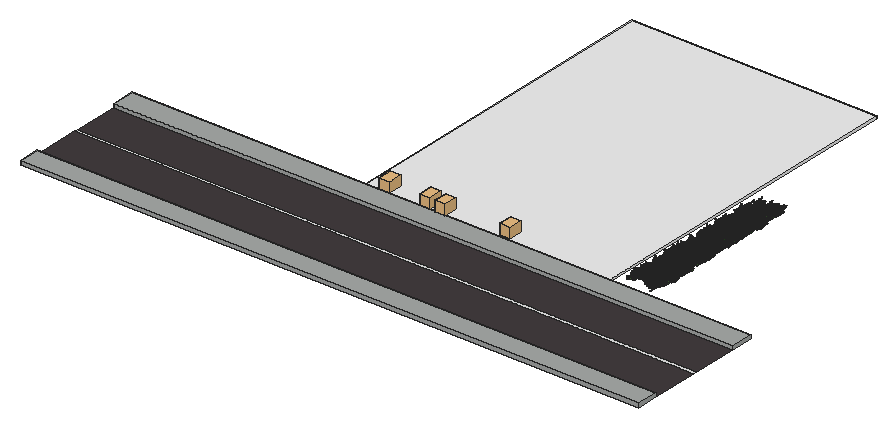
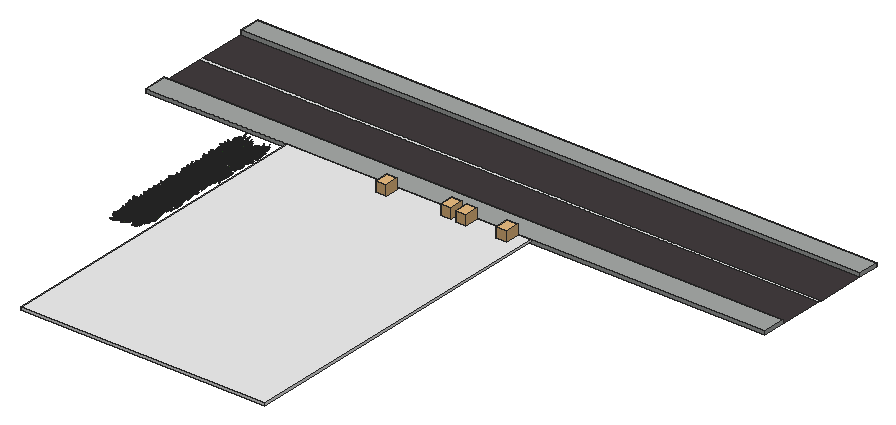
# SketchUp Ruby script. Lengths in inches.
U = 1.inch
M = Sketchup.active_model
def pt(a) = Geom::Point3d.new(a.map { |v| v * U })
def face(e, loops, mat)
  f = e.add_face(loops[0].map { |a| pt(a) })
  loops[1..].each { |l| e.add_face(l.map { |a| pt(a) }).erase! }
  f.material = f.back_material = mat if mat
  f
end
# faces: each face lists its corners as indices into pts; further lists are holes
def faces(e, pts, list, mat = nil) = list.each { |f| face(e, (f[0].is_a?(Array) ? f : [f]).map { |l| l.map { |i| pts[i] } }, mat) }
# xy, xz, yz: faces in a plane at the given z, y or x. An outline is a flat list of corners, or four numbers for a rectangle; further outlines are holes
def ring(l) = l.size == 4 ? [[l[0], l[1]], [l[2], l[1]], [l[2], l[3]], [l[0], l[3]]] : l.each_slice(2).to_a
def flat(e, list, mat, &to3) = list.each { |f| face(e, (f[0].is_a?(Array) ? f : [f]).map { |l| ring(l).map { |u, v| to3.(u, v) } }, mat) }
def xy(e, z, list, mat = nil) = flat(e, list, mat) { |x, y| [x, y, z] }
def xz(e, y, list, mat = nil) = flat(e, list, mat) { |x, z| [x, y, z] }
def yz(e, x, list, mat = nil) = flat(e, list, mat) { |y, z| [x, y, z] }
def lines(e, pts, list) = list.each { |a, b| e.add_line(pt(pts[a]), pt(pts[b])) }
# prism: a flat outline (further loops are holes) pulled along v
def prism(e, loops, v, mat = nil)
  f = face(e, loops, mat); d = Geom::Vector3d.new(v.map { |x| x * U })
  f.pushpull(f.normal.samedirection?(d) ? d.length : -d.length)
end
def box(e, o, s, mat = nil) = prism(e, [[o, [o[0] + s[0], o[1], o[2]], [o[0] + s[0], o[1] + s[1], o[2]], [o[0], o[1] + s[1], o[2]]]], [0, 0, s[2]], mat)
def at(x, y, z, deg = 0) = Geom::Transformation.translation(pt([x, y, z])) * Geom::Transformation.rotation(ORIGIN, Z_AXIS, deg.degrees)
def axes(o, x, y, z) = Geom::Transformation.new([*x, 0, *y, 0, *z, 0, *pt(o).to_a, 1])
def part(name) = M.definitions.add(name)
# library, detail: a bought-in or finely detailed component or shape, given as its bounding box
def library(name, o, s) = part(name).tap { |d| box(d.entities, o, s) }
def detail(e, o, s) = box(e.add_group.entities, o, s)
def put(e, d, t, mat = nil) = e.add_instance(d, t).tap { |i| i.material = mat if mat }
def group(e, t, mat = nil) = e.add_group.tap { |g| g.transformation = t; g.material = mat if mat }.entities
root = M.entities
M.materials.add("Material10").color = [48, 90, 38]
M.materials.add("Material11").color = [68, 110, 48]
M.materials.add("Material12").color = [48, 90, 48]
M.materials.add("Material13").color = [58, 110, 58]
M.materials.add("Material14").color = [58, 90, 38]
M.materials.add("Material15").color = [68, 100, 58]
M.materials.add("Material16").color = [48, 100, 38]
M.materials.add("Material9").color = [68, 110, 58]
M.materials.add("Tiles Marble White 03 180cm\#1").color = [241, 241, 241]
M.materials.add("[Asphalt_New]").color = [67, 60, 62]
M.materials.add("[Color_001]1").color = [226, 226, 226]
M.materials.add("[Concrete_Form_4x8]").color = [167, 170, 168]
c1 = library("Plant 260 031 02",[-5.66,-10.61,-5.67],[17.04,23.05,21.91])
c2 = part("组\#1")
xy(c2.entities,0,[[37.85,0,110.93,506],[116.54,0,195.23,506]],"[Asphalt_New]")
xy(c2.entities,0,[[110.93,0,116.54,506]],"[Color_001]1")
xy(c2.entities,6.25,[[0,0,37.85,506],[195.23,0,229.75,506]],"[Concrete_Form_4x8]")
xz(c2.entities,0,[[0,0,37.85,6.25],[195.23,0,229.75,6.25]],"[Concrete_Form_4x8]")
xz(c2.entities,506,[[0,0,37.85,6.25],[195.23,0,229.75,6.25]],"[Concrete_Form_4x8]")
yz(c2.entities,0,[[0,0,506,6.25]],"[Concrete_Form_4x8]")
yz(c2.entities,37.85,[[0,0,506,6.25]],"[Concrete_Form_4x8]")
yz(c2.entities,195.23,[[0,0,506,6.25]],"[Concrete_Form_4x8]")
yz(c2.entities,229.75,[[0,0,506,6.25]],"[Concrete_Form_4x8]")
c3 = part("grass00")
p = [[-0.6875,0.15,0],[-0.56,0.08,5.52],[-0.04,0.03,2.76],[0.48,-0.02,0],[0.35,-0.02,5.52],[-0.1,-0.14,5.52],
  [-0.12,0.65,8.37],[-0.42,0.65,8.37]]
faces(c3.entities,p,[[0,1,2,3],[3,2,4],[1,5,2],[5,4,2],[1,6,5],[4,5,6],[7,6,1]])
c4 = part("Group16\#1")
put(c4.entities,c3,axes([1.44,-0.61,-0.01],[0.05352,0.12609,0],[-0.10704,0.04543,0.07239],[0.06664,-0.02828,0.11628]),"Material12")
put(c4.entities,c3,axes([0.76,-0.15,-0.01],[0.04676,0.24062,0],[-0.23162,0.04501,0.06642],[0.0652,-0.01267,0.23595]),"Material9")
put(c4.entities,c3,axes([0.79,0.01,-0.01],[-0.00606,0.34651,0],[-0.34381,-0.00602,0.0432],[0.04319,0.00076,0.34386]))
put(c4.entities,c3,axes([1,0.23,-0.01],[-0.07192,0.31144,0],[-0.28722,-0.06632,0.1236],[0.12043,0.02781,0.29478]),"Material11")
put(c4.entities,c3,axes([1.66,0.77,-0.01],[-0.13828,0.29651,0],[-0.21551,-0.1005,0.22471],[0.20365,0.09498,0.23779]),"Material16")
put(c4.entities,c3,axes([0.6875,0.52,-0.01],[-0.18126,0.24051,0],[-0.22746,-0.17142,0.09788],[0.07817,0.05891,0.28481]),"Material11")
put(c4.entities,c3,axes([0.68,0.78,-0.01],[-0.215,0.18688,0],[-0.12385,-0.14248,0.21334],[0.13995,0.16101,0.18878]),"Material9")
put(c4.entities,c3,axes([0.56,1,-0.01],[-0.13756,0.07624,0],[-0.06159,-0.11112,0.0927],[0.04494,0.08108,0.12705]),"Material11")
put(c4.entities,c3,axes([0.2,0.64,-0.01],[-0.23729,0.07254,0],[-0.05711,-0.18681,0.153],[0.04473,0.14632,0.19535]),"Material16")
put(c4.entities,c3,axes([0.0625,0.72,-0.01],[-0.28874,0.02525,0],[-0.02179,-0.24916,0.14647],[0.01276,0.14591,0.25012]),"Material9")
put(c4.entities,c3,axes([-0.08,0.62,-0.01],[-0.34089,-0.04187,0],[0.03255,-0.26504,0.216],[-0.02633,0.21439,0.26703]),"Material16")
put(c4.entities,c3,axes([-0.34,0.98,-0.01],[-0.14314,-0.0493,0],[0.04397,-0.12769,0.06843],[-0.02228,0.0647,0.13505]),"Material16")
put(c4.entities,c3,axes([-0.87,1.45,-0.01],[-0.23488,-0.14114,0],[0.13761,-0.22901,0.06087],[-0.03135,0.05217,0.26717]))
put(c4.entities,c3,axes([-0.72,0.77,-0.01],[-0.14208,-0.13251,0],[0.07209,-0.0773,0.16301],[-0.11118,0.11922,0.1057]),"Material16")
put(c4.entities,c3,axes([-0.62,0.43,-0.01],[-0.14845,-0.21203,0],[0.18654,-0.13061,0.12304],[-0.10079,0.07057,0.22772]),"Material9")
put(c4.entities,c3,axes([-0.68,0.29,-0.01],[-0.13639,-0.32136,0],[0.31723,-0.13464,0.05579],[-0.05136,0.0218,0.34462]),"Material10")
put(c4.entities,c3,axes([-0.64,0.125,-0.01],[-0.0458,-0.23569,0],[0.22124,-0.043,0.08276],[-0.08124,0.01579,0.22538]),"Material13")
put(c4.entities,c3,axes([-1.6,-0.03,-0.01],[0.00576,-0.32897,0],[0.27526,0.00482,0.18018],[-0.18015,-0.00315,0.2753]),"Material11")
put(c4.entities,c3,axes([-1.36,-0.31,-0.01],[0.05718,-0.24765,0],[0.18172,0.04196,0.17267],[-0.16825,-0.03885,0.1865]),"Material16")
put(c4.entities,c3,axes([-1.54,-0.72,-0.01],[0.06537,-0.14017,0],[0.13555,0.06321,0.03939],[-0.0357,-0.01665,0.14956]))
put(c4.entities,c3,axes([-1.19,-0.9,-0.01],[0.09597,-0.12735,0],[0.11214,0.08451,0.07557],[-0.06035,-0.04548,0.14042]),"Material15")
put(c4.entities,c3,axes([-0.47,-0.54,-0.01],[0.11588,-0.10072,0],[0.0618,0.0711,0.12124],[-0.07953,-0.0915,0.0942]))
put(c4.entities,c3,axes([-0.47,-0.84,-0.01],[0.11927,-0.0661,0],[0.06603,0.11913,0.00646],[-0.00313,-0.00565,0.13621]),"Material11")
put(c4.entities,c3,axes([-0.38,-1.24,-0.01],[0.28037,-0.08571,0],[0.0618,0.20215,0.20315],[-0.05939,-0.19428,0.21139]),"Material15")
put(c4.entities,c3,axes([-0.06,-0.66,-0.01],[0.22719,-0.01987,0],[0.01247,0.14255,0.17758],[-0.01547,-0.17691,0.1431]),"Material14")
put(c4.entities,c3,axes([0.11,-0.89,-0.01],[0.14882,0.01828,0],[-0.01058,0.08611,0.12229],[0.01491,-0.12138,0.08676]),"Material12")
put(c4.entities,c3,axes([0.25,-0.72,-0.01],[0.20481,0.07053,0],[-0.06206,0.18022,0.10291],[0.03351,-0.0973,0.1906]),"Material12")
put(c4.entities,c3,axes([0.85,-1.42,-0.01],[0.16481,0.09904,0],[-0.09472,0.15762,0.05616],[0.02893,-0.04814,0.18389]),"Material11")
put(c4.entities,c3,axes([1.01,-1.09,-0.01],[0.21858,0.20385,0],[-0.17495,0.1876,0.15339],[0.10462,-0.11218,0.25652]),"Material16")
put(c4.entities,c3,axes([1.01,-0.71,-0.01],[0.08733,0.12473,0],[-0.06445,0.04512,0.13037],[0.1068,-0.07477,0.07867]),"Material12")
c5 = part("Group15\#1")
put(c5.entities,c4,at(0,0,0))
c6 = part("3darcstudiotree_grass00\#1")
put(c6.entities,c5,at(0,0,0))
put(root,c1,at(411.73,241.75,16.75))
put(root,c1,at(479.07,241.3,16.75))
put(root,c1,at(505.1,239.68,16.75))
put(root,c2,axes([0,229.75,10.5],[0,-1,0],[2.0148,0,0],[0,0,1]))
g1 = group(root,at(420.73,303.57,12.75))
box(g1,[-36,-73.82,0],[402,549.37,4],"Tiles Marble White 03 180cm\#1")
put(root,c1,at(607.78,244.29,16.75))
put(root,c6,axes([800.67,339.93,12.99],[-0.98849,-6.07727,0],[3.06022,-2.60089,-0.02925],[0.10433,-0.08867,1.7044]))
put(root,c6,axes([800.7,291.18,12.99],[-3.25842,-2.83889,0],[0.88861,-5.32937,-0.04688],[0.07754,-0.46503,1.58936]))
put(root,c6,axes([800.98,446.97,12.99],[-1.08167,-7.23461,0],[2.82341,-2.20577,-0.03013],[0.10703,-0.08362,1.53631]))
put(root,c6,axes([800.78,348.7,12.99],[-1.3715,5.90605,0],[-2.459,-2.98374,-0.02935],[-0.08981,-0.10898,1.32321]))
put(root,c6,axes([800.82,311.72,12.99],[2.39933,-0.88558,0],[0.42391,6.00129,-0.03713],[0.0226,0.31997,1.39317]))
put(root,c6,axes([801.01,271.4,12.99],[1.11384,7.00141,0],[-2.3963,1.99197,-0.03897],[-0.1605,0.13341,1.53286]))
put(root,c6,axes([802.48,486.76,12.99],[0.27051,-7.1157,0],[3.04279,0.60444,-0.03115],[0.11632,0.02311,1.5702]))
put(root,c6,axes([803.05,273.92,12.99],[1.68247,-4.28756,0],[2.47865,5.08226,-0.03873],[0.1199,0.24584,1.89965]))
put(root,c6,axes([803.99,418.8,12.99],[1.17417,-7.15261,0],[2.37757,2.03942,-0.02337],[0.10494,0.09002,1.67088]))
put(root,c6,axes([803.49,282.77,12.99],[0.14761,6.20223,0],[-2.49222,0.30993,-0.03311],[-0.1396,0.01736,1.44579]))
put(root,c6,axes([804.68,413.44,12.99],[-2.29924,4.62436,0],[-1.90032,-4.937,-0.02195],[-0.06693,-0.17388,1.82186]))
put(root,c6,axes([805.44,366.33,12.99],[-2.97813,-1.40056,0],[0.64267,-7.14054,-0.02294],[0.01821,-0.20232,1.72347]))
put(root,c6,axes([804.71,346.85,12.99],[2.49242,-3.45573,0],[1.7696,6.66902,-0.03972],[0.07236,0.27271,1.6444]))
put(root,c6,axes([804.3,395.07,12.99],[2.7147,4.27072,0],[-1.80498,5.99513,-0.05897],[-0.14635,0.48608,1.91169]))
put(root,c6,axes([805.35,357.75,12.99],[-2.03898,5.04396,0],[-2.47769,-5.23352,-0.01856],[-0.05439,-0.11488,1.84646]))
put(root,c6,axes([805.07,262.63,12.99],[2.98145,-0.50513,0],[0.21055,6.4935,-0.02045],[0.00697,0.21501,1.8024]))
put(root,c6,axes([806.57,467.15,12.99],[-0.75501,-6.88565,0],[2.48437,-1.4234,-0.0349],[0.17754,-0.10172,1.84282]))
put(root,c6,axes([807.58,414.25,12.99],[-1.68018,-4.94064,0],[2.1447,-3.81105,-0.04864],[0.19458,-0.34576,1.88819]))
put(root,c6,axes([807.57,335.99,12.99],[-0.20197,-5.97763,0],[2.99307,-0.52842,-0.04603],[0.17968,-0.03172,1.61216]))
put(root,c6,axes([807.93,424.48,12.99],[-3.12761,-0.88156,0],[0.3332,-6.17695,-0.03319],[0.01691,-0.31352,1.55524]))
put(root,c6,axes([808.16,484.11,12.99],[-0.99694,-6.52822,0],[3.15637,-2.51865,-0.05387],[0.16231,-0.12952,1.46363]))
put(root,c6,axes([807.17,373.95,12.99],[2.63554,-0.55768,0],[0.2785,6.87733,-0.05657],[0.01882,0.46468,1.49576]))
put(root,c6,axes([808.32,438,12.99],[-2.32089,-3.24237,0],[1.49534,-5.59289,-0.04274],[0.09418,-0.35224,1.66217]))
put(root,c6,axes([807.77,448.18,12.99],[-0.45873,6.51223,0],[-2.66489,-0.98087,-0.03829],[-0.17369,-0.06393,1.70109]))
put(root,c6,axes([808.8,402.28,12.99],[-0.66116,-7.15231,0],[3.12813,-1.51095,-0.02196],[0.08817,-0.04259,1.79942]))
put(root,c6,axes([809.1,359.21,12.99],[-3.21408,-1.17783,0],[0.46153,-6.58082,-0.05495],[0.03492,-0.49786,1.60563]))
put(root,c6,axes([808.84,503.35,12.99],[1.24877,-5.5627,0],[2.72354,3.19474,-0.0206],[0.07656,0.08981,1.75423]))
put(root,c6,axes([808.12,349.19,12.99],[1.31042,5.62084,0],[-2.40949,2.93521,-0.05193],[-0.22679,0.27628,1.85357]))
put(root,c6,axes([809.27,427.29,12.99],[0.39081,-6.30576,0],[2.59761,0.84122,-0.02485],[0.13497,0.04371,1.97391]))
put(root,c6,axes([809.24,289.6,12.99],[-1.24855,7.36062,0],[-2.95077,-2.61536,-0.03012],[-0.11789,-0.10449,1.82227]))
put(root,c6,axes([809.14,475.84,12.99],[1.94397,4.23046,0],[-2.00085,4.80421,-0.04733],[-0.10808,0.2595,1.31836]))
put(root,c6,axes([809.4,315.22,12.99],[1.81122,6.51683,0],[-2.34506,3.4056,-0.05376],[-0.20203,0.2934,1.69687]))
put(root,c6,axes([810.82,299.03,12.99],[-2.35732,-4.30403,0],[1.59602,-4.56758,-0.04095],[0.12835,-0.36732,1.76156]))
put(root,c6,axes([811.1,441.46,12.99],[-1.06173,6.81827,0],[-2.83321,-2.30528,-0.05045],[-0.18809,-0.15304,1.63245]))
put(root,c6,axes([810.82,448.49,12.99],[1.33722,6.52276,0],[-2.56931,2.75228,-0.0367],[-0.17016,0.18228,1.99296]))
put(root,c6,axes([811.93,272.2,12.99],[-2.43072,-0.26359,0],[0.12868,-6.20017,-0.03298],[0.00788,-0.37965,1.87797]))
put(root,c6,axes([812.05,486.26,12.99],[-0.28872,-6.59919,0],[3.07918,-0.70393,-0.04439],[0.1451,-0.03317,1.39437]))
put(root,c6,axes([812.05,372.78,12.99],[-2.52267,-1.45098,0],[0.6301,-5.72418,-0.02412],[0.0269,-0.24434,1.61843]))
put(root,c6,axes([811.96,408.8,12.99],[-2.43865,3.44906,0],[-1.64275,-6.06912,-0.03047],[-0.05197,-0.19201,1.38852]))
put(root,c6,axes([811.48,479.91,12.99],[3.0655,-2.19528,0],[0.96462,7.03842,-0.0458],[0.05493,0.40081,1.7756]))
put(root,c6,axes([811.24,286.83,12.99],[2.42292,5.76115,0],[-1.8644,4.09707,-0.03508],[-0.11405,0.25063,1.59982]))
put(root,c6,axes([812.07,278.9375,12.99],[1.67096,-5.47383,0],[2.37534,3.78884,-0.05108],[0.18896,0.3014,1.79238]))
put(root,c6,axes([811.78,429.89,12.99],[-1.17862,5.63021,0],[-2.88982,-3.16101,-0.03408],[-0.09497,-0.10388,1.35762]))
put(root,c6,axes([812.84,418.5625,12.99],[-0.22622,-6.9338,0],[3.33092,-0.56785,-0.02024],[0.08123,-0.01385,1.84439]))
put(root,c6,axes([812.42,495.47,12.99],[2.21202,-5.60133,0],[2.54118,5.24369,-0.0538],[0.11673,0.24088,1.37259]))
put(root,c6,axes([812.81,344.54,12.99],[-1.98571,5.23753,0],[-2.13766,-4.2348,-0.03703],[-0.1146,-0.22703,1.58908]))
put(root,c6,axes([812.24,456.87,12.99],[0.79567,6.14666,0],[-3.11802,2.10902,-0.04809],[-0.14133,0.0956,1.36712]))
put(root,c6,axes([813.4,394.8,12.99],[2.47868,-2.12288,0],[0.90034,5.49294,-0.02122],[0.03978,0.2427,1.88089]))
put(root,c6,axes([814.86,448.8,12.99],[-2.3446,-1.56119,0],[0.96027,-7.5355,-0.03129],[0.03426,-0.26886,1.8441]))
put(root,c6,axes([815.66,289.4,12.99],[-2.01079,-4.32886,0],[2.15818,-5.23823,-0.03536],[0.10109,-0.24536,1.8008]))
put(root,c6,axes([814.9,368.54,12.99],[-0.72251,7.60275,0],[-2.80101,-1.39088,-0.03052],[-0.10543,-0.05235,1.38983]))
put(root,c6,axes([814.87,410.37,12.99],[-0.62691,6.10742,0],[-2.93793,-1.57578,-0.03302],[-0.11697,-0.06274,1.5061]))
put(root,c6,axes([815.87,284.22,12.99],[1.28541,-7.35574,0],[2.62364,2.39566,-0.05078],[0.21024,0.19197,1.72798]))
put(root,c6,axes([815.28,271.93,12.99],[0.93965,5.53656,0],[-2.59756,2.30353,-0.02781],[-0.10678,0.09469,1.57422]))
put(root,c6,axes([815.47,317.37,12.99],[2.51332,0.19657,0],[-0.11442,7.6442,-0.02332],[-0.00314,0.20995,1.80921]))
put(root,c6,axes([815.29,470.8,12.99],[1.0999,5.70723,0],[-2.59262,2.61079,-0.02705],[-0.09815,0.09884,1.54111]))
put(root,c6,axes([817.08,305.77,12.99],[-1.20299,-5.03385,0],[2.72849,-3.40713,-0.05959],[0.16003,-0.19984,1.30502]))
put(root,c6,axes([816.5,430.53,12.99],[1.31185,-4.97646,0],[2.11718,2.91626,-0.04784],[0.21048,0.28992,1.7418]))
put(root,c6,axes([816.1,422.85,12.99],[0.16456,7.31733,0],[-3.11559,0.36612,-0.0387],[-0.15466,0.01817,1.71236]))
put(root,c6,axes([815.98,373.42,12.99],[1.03995,6.32855,0],[-3.24295,2.78455,-0.05425],[-0.18431,0.15826,1.72469]))
put(root,c6,axes([816.29,497.62,12.99],[2.76605,-1.75518,0],[0.75789,6.24093,-0.05393],[0.0673,0.55416,1.81331]))
put(root,c6,axes([816.83,339.07,12.99],[-0.70332,7.47702,0],[-2.7387,-1.34609,-0.03186],[-0.1588,-0.07805,1.95913]))
put(root,c6,axes([817.6,478.36,12.99],[2.41352,-1.75969,0],[1.02756,7.3642,-0.05774],[0.07229,0.51811,1.91123]))
put(root,c6,axes([817.64,330.62,12.99],[3.37945,0.43102,0],[-0.14532,5.9535,-0.03032],[-0.00727,0.29784,1.54015]))
put(root,c6,axes([819.5,327.62,12.99],[-1.60721,-5.62738,0],[2.90847,-4.34044,-0.04707],[0.1152,-0.17193,1.39282]))
put(root,c6,axes([819.24,289.91,12.99],[-2.47982,0.43946,0],[-0.21468,-6.33001,-0.03359],[-0.01335,-0.39362,1.95875]))
put(root,c6,axes([818.82,274.38,12.99],[2.90022,-1.64439,0],[0.76036,7.00726,-0.04456],[0.03552,0.32738,1.43455]))
put(root,c6,axes([819.93,374.12,12.99],[0.44477,-5.91225,0],[2.87147,1.12875,-0.05034],[0.22005,0.0865,1.77282]))
put(root,c6,axes([819.45,281.14,12.99],[2.90811,-3.84565,0],[1.47455,5.82647,-0.042],[0.08136,0.32147,1.56273]))
put(root,c6,axes([819.58,493.84,12.99],[-0.82136,5.5989,0],[-2.45056,-1.87847,-0.03292],[-0.17046,-0.13067,1.93659]))
put(root,c6,axes([820.58,429.28,12.99],[-1.12864,-5.67163,0],[2.36562,-2.45979,-0.03768],[0.17047,-0.17726,1.77164]))
put(root,c6,axes([819.91,452.42,12.99],[-0.76606,6.14849,0],[-3.01347,-1.96186,-0.05457],[-0.16844,-0.10966,1.37935]))
put(root,c6,axes([820.83,458.83,12.99],[-2.64198,-0.01413,0],[0.00691,-6.75381,-0.04252],[0.00042,-0.41186,1.71753]))
put(root,c6,axes([820.62,442.89,12.99],[1.08338,-7.38088,0],[2.98288,2.28778,-0.04434],[0.18837,0.14447,1.93394]))
put(root,c6,axes([820.1,483.2,12.99],[0.63272,5.75495,0],[-3.24747,1.8656,-0.04255],[-0.14077,0.08087,1.5668]))
put(root,c6,axes([820.26,409,12.99],[-0.06557,6.27444,0],[-3.01984,-0.1649,-0.0357],[-0.12361,-0.00675,1.43525]))
put(root,c6,axes([820.75,352.63,12.99],[-1.14002,6.6101,0],[-2.92889,-2.63945,-0.03242],[-0.13715,-0.1236,1.96368]))
put(root,c6,axes([820.98,464.85,12.99],[2.21805,-5.1578,0],[1.9196,4.31342,-0.02297],[0.07437,0.16711,1.67632]))
put(root,c6,axes([821.73,344.23,12.99],[-3.00149,-1.29582,0],[0.62931,-7.61662,-0.03943],[0.0254,-0.30742,1.61444]))
put(root,c6,axes([821.25,385.67,12.99],[3.35583,0.90244,0],[-0.36623,7.11602,-0.02625],[-0.01403,0.27269,1.96735]))
put(root,c6,axes([823.05,428.82,12.99],[1.48515,-4.64439,0],[2.70372,4.5176,-0.0361],[0.11436,0.19109,1.80295]))
put(root,c6,axes([823.24,386.95,12.99],[2.79596,-0.85761,0],[0.37281,6.35086,-0.04419],[0.02295,0.39103,1.50171]))
put(root,c6,axes([823.15,272.84,12.99],[2.3384,1.9666,0],[-1.12017,6.95972,-0.05896],[-0.0889,0.55232,1.94308]))
put(root,c6,axes([824.01,495.11,12.99],[0.57994,-6.73652,0],[2.86103,1.28699,-0.05061],[0.24221,0.10895,1.95081]))
put(root,c6,axes([824.42,404.06,12.99],[-3.14593,0.19669,0],[-0.0805,-6.72751,-0.04984],[-0.00504,-0.42161,1.49526]))
put(root,c6,axes([824.4,409.32,12.99],[0.49075,-6.40582,0],[3.38111,1.35347,-0.04237],[0.17115,0.06851,1.93074]))
put(root,c6,axes([823.99,377.41,12.99],[-1.60507,4.37133,0],[-2.1394,-4.10464,-0.02769],[-0.08294,-0.15912,1.49833]))
put(root,c6,axes([824.06,343.74,12.99],[-0.89948,6.8666,0],[-2.40007,-1.64278,-0.04102],[-0.19098,-0.13072,1.67021]))
put(root,c6,axes([824.46,338.08,12.99],[-2.39967,1.77823,0],[-0.84177,-5.93558,-0.02033],[-0.03221,-0.22713,1.92362]))
put(root,c6,axes([824.9,504.92,12.99],[1.19643,-5.17375,0],[2.94616,3.55995,-0.05061],[0.19141,0.23129,1.95538]))
put(root,c6,axes([825.47,278.9,12.99],[-3.25043,-1.79048,0],[0.7178,-6.80898,-0.03666],[0.0266,-0.2523,1.30149]))
put(root,c6,axes([825.57,448.05,12.99],[0.70032,-6.09553,0],[2.75723,1.65525,-0.03356],[0.13373,0.08028,1.61101]))
put(root,c6,axes([824.82,318.11,12.99],[2.9474,-0.64535,0],[0.26292,6.27452,-0.02913],[0.01462,0.34879,1.9903]))
put(root,c6,axes([825.83,392.66,12.99],[0.08346,-7.87109,0],[3.34792,0.1855,-0.04883],[0.16939,0.00939,1.59403]))
put(root,c6,axes([825.17,438.74,12.99],[3.21665,-2.7044,0],[1.05278,6.54301,-0.01984],[0.03125,0.19424,1.90869]))
put(root,c6,axes([827.4,300.69,12.99],[0.04219,-5.7063,0],[3.45233,0.13336,-0.02351],[0.08008,0.00309,1.61343]))
put(root,c6,axes([826.95,334.32,12.99],[1.89108,-4.73646,0],[2.37989,4.96499,-0.03913],[0.10141,0.21157,1.55084]))
put(root,c6,axes([827.46,410.77,12.99],[-3.44336,1.49211,0],[-0.55386,-6.67865,-0.04366],[-0.03407,-0.41081,1.70895]))
put(root,c6,axes([827.6875,376.23,12.99],[-3.3483,-0.40679,0],[0.16926,-7.27961,-0.02618],[0.00551,-0.23685,1.73378]))
put(root,c6,axes([827.94,458.25,12.99],[-2.66261,-3.09457,0],[1.21392,-5.45761,-0.05096],[0.10103,-0.45421,1.60728]))
put(root,c6,axes([828.45,308.6875,12.99],[-2.3271,-5.73934,0],[2.28196,-4.83467,-0.01903],[0.06279,-0.13303,1.91973]))
put(root,c6,axes([828.06,496.02,12.99],[1.46618,-4.65732,0],[2.76551,4.54916,-0.05142],[0.17625,0.28992,1.97373]))
put(root,c6,axes([827.39,365.65,12.99],[1.46208,4.72048,0],[-2.56718,4.15477,-0.06047],[-0.15344,0.24833,1.34144]))
put(root,c6,axes([828.67,469.4375,12.99],[-0.88269,-5.76052,0],[2.35523,-1.88576,-0.02961],[0.10967,-0.08781,1.34337]))
put(root,c6,axes([828.02,404.45,12.99],[2.19606,-2.73219,0],[1.30755,5.49159,-0.04084],[0.10103,0.42434,1.94165]))
put(root,c6,axes([829.23,421.82,12.99],[-2.01827,-3.48748,0],[1.88505,-5.70027,-0.03674],[0.08372,-0.25316,1.62045]))
put(root,c6,axes([829.22,287.63,12.99],[-3.34809,0.09991,0],[-0.04255,-7.45093,-0.02897],[-0.00121,-0.21243,1.4344]))
put(root,c6,axes([828.375,483.74,12.99],[2.57024,-1.2356,0],[0.65378,7.10617,-0.04208],[0.02654,0.28851,1.3356]))
put(root,c6,axes([828.3125,274.93,12.99],[2.34968,4.58189,0],[-2.19552,5.8831,-0.05603],[-0.14074,0.37713,1.79617]))
put(root,c6,axes([829.54,442.75,12.99],[1.14969,-6.54059,0],[3.15217,2.89521,-0.03894],[0.15163,0.13927,1.95573]))
put(root,c6,axes([829.42,395.61,12.99],[1.62972,-6.70188,0],[2.2894,2.90899,-0.02727],[0.09591,0.12187,1.44583]))
put(root,c6,axes([829.32,264.82,12.99],[2.77012,2.08951,0],[-0.77702,5.38259,-0.0401],[-0.06244,0.43256,1.69032]))
put(root,c6,axes([831.08,422.73,12.99],[-3.36606,1.19187,0],[-0.50092,-7.39208,-0.03016],[-0.01674,-0.24697,1.62739]))
put(root,c6,axes([831.375,270.125,12.99],[-2.52074,1.42331,0],[-0.64151,-5.93654,-0.03348],[-0.03327,-0.30786,1.52035]))
put(root,c6,axes([832.29,475.09,12.99],[-3.27375,-1.41697,0],[0.56283,-6.79472,-0.02653],[0.02016,-0.24334,1.69452]))
put(root,c6,axes([832.77,319.14,12.99],[-0.71606,-7.27219,0],[2.95093,-1.51827,-0.03143],[0.11287,-0.05807,1.52743]))
put(root,c6,axes([832.89,484.05,12.99],[-2.55654,-1.32482,0],[0.6468,-6.5218,-0.03754],[0.04019,-0.40529,1.94323]))
put(root,c6,axes([832.67,324.84,12.99],[-0.3249,-6.84497,0],[2.61307,-0.6481,-0.05057],[0.24759,-0.06141,1.77563]))
put(root,c6,axes([831.92,383.67,12.99],[2.28145,2.83772,0],[-1.30496,5.48204,-0.04213],[-0.07295,0.30646,1.35679]))
put(root,c6,axes([832.1,355.6,12.99],[2.65726,4.78075,0],[-1.95968,5.69151,-0.01986],[-0.05463,0.15866,1.93312]))
put(root,c6,axes([832.71,503.55,12.99],[2.90532,0.03051,0],[-0.01147,5.70878,-0.03904],[-0.00097,0.48249,1.85207]))
put(root,c6,axes([833.45,343.03,12.99],[1.45867,-7.28419,0],[2.5237,2.6407,-0.04178],[0.16201,0.16952,1.62381]))
put(root,c6,axes([832.82,399.47,12.99],[2.4435,3.96341,0],[-1.87885,6.05257,-0.05586],[-0.11091,0.35728,1.52805]))
put(root,c6,axes([833.51,468.47,12.99],[2.28966,-1.89276,0],[1.03348,6.53259,-0.04794],[0.05324,0.33652,1.36124]))
put(root,c6,axes([834.0625,461.92,12.99],[2.21452,-3.37986,0],[1.80124,6.16677,-0.03164],[0.07505,0.25694,1.90074]))
put(root,c6,axes([833.54,451.42,12.99],[1.27497,7.41001,0],[-2.91745,2.62294,-0.01805],[-0.07436,0.06685,1.90362]))
put(root,c6,axes([833.95,437.6875,12.99],[3.28738,-2.27576,0],[0.93503,7.05752,-0.03542],[0.03342,0.25223,1.44036]))
put(root,c6,axes([835.22,439.19,12.99],[-3.06604,0.56659,0],[-0.20624,-5.83149,-0.02584],[-0.01034,-0.29231,1.74304]))
put(root,c6,axes([835.14,468.41,12.99],[1.76576,-3.84655,0],[1.76477,4.23305,-0.03437],[0.11275,0.27045,1.66865]))
put(root,c6,axes([835.65,486.03,12.99],[0.28434,-7.40273,0],[2.77399,0.55675,-0.02351],[0.1012,0.02031,1.65028]))
put(root,c6,axes([836.84,289.66,12.99],[-2.3348,-1.65014,0],[0.9334,-6.90079,-0.02785],[0.03444,-0.25462,1.81462]))
put(root,c6,axes([836.35,309.56,12.99],[-1.11841,5.19115,0],[-2.48378,-2.79613,-0.03193],[-0.1283,-0.14443,1.70102]))
put(root,c6,axes([837.19,336.92,12.99],[-2.77442,0.55042,0],[-0.21198,-5.58304,-0.03872],[-0.01779,-0.46848,1.78675]))
put(root,c6,axes([836.25,504.96,12.99],[2.43451,2.43826,0],[-1.37998,7.19963,-0.0492],[-0.06463,0.3372,1.54416]))
put(root,c6,axes([836.49,318.17,12.99],[2.37812,1.75017,0],[-0.85893,6.09842,-0.048],[-0.07035,0.49946,1.83855]))
put(root,c6,axes([837.52,476.84,12.99],[0.73631,-5.3027,0],[3.29322,2.3894,-0.04397],[0.12671,0.09193,1.43296]))
put(root,c6,axes([836.6875,420.89,12.99],[0.94107,7.03286,0],[-3.28145,2.29435,-0.03143],[-0.09131,0.06384,1.42994]))
put(root,c6,axes([837.22,389.93,12.99],[2.74309,-3.90813,0],[1.56596,5.74323,-0.04378],[0.10229,0.37515,1.79394]))
put(root,c6,axes([836.92,356.41,12.99],[0.54691,6.82765,0],[-3.28718,1.37585,-0.04305],[-0.169,0.07073,1.82947]))
put(root,c6,axes([837.04,284.04,12.99],[2.34307,2.00121,0],[-1.05989,6.48424,-0.02415],[-0.03918,0.23972,1.92547]))
put(root,c6,axes([837.25,372.94,12.99],[0.42922,7.58732,0],[-2.88779,0.85362,-0.04685],[-0.19486,0.0576,1.67517]))
put(root,c6,axes([838.13,429.08,12.99],[0.7602,-5.62584,0],[2.50138,1.76613,-0.03395],[0.13629,0.09623,1.50895]))
put(root,c6,axes([837.42,448.3125,12.99],[2.60951,5.13082,0],[-1.93207,5.13453,-0.04839],[-0.11468,0.30476,1.47711]))
put(root,c6,axes([839.7,347.3,12.99],[-1.80025,-4.99335,0],[1.95168,-3.67666,-0.03867],[0.12878,-0.2426,1.49724]))
put(root,c6,axes([839.98,283.9375,12.99],[-2.17621,-2.64164,0],[1.45611,-6.26796,-0.05452],[0.0843,-0.36287,1.404]))
put(root,c6,axes([840.04,263.39,12.99],[0.41364,-7.76369,0],[2.81089,0.78254,-0.0324],[0.12251,0.03411,1.47946]))
put(root,c6,axes([840.57,314.91,12.99],[-0.32018,-7.31674,0],[2.81539,-0.64376,-0.05423],[0.23614,-0.05399,1.69842]))
put(root,c6,axes([840.63,330.51,12.99],[-2.47658,3.74512,0],[-1.53429,-5.30151,-0.03289],[-0.07404,-0.25584,1.55622]))
put(root,c6,axes([841.17,353.07,12.99],[-2.06374,-4.42299,0],[1.67217,-4.07684,-0.04465],[0.15651,-0.38158,1.71883]))
put(root,c6,axes([841.49,269.08,12.99],[-2.94351,-3.72862,0],[1.6201,-6.6829,-0.02403],[0.04879,-0.20124,1.92026]))
put(root,c6,axes([841.75,289.98,12.99],[-1.65176,-4.19252,0],[2.05027,-4.22073,-0.04825],[0.17559,-0.36148,1.85346]))
put(root,c6,axes([841.22,447.14,12.99],[-1.97291,5.66606,0],[-2.22162,-4.04204,-0.02078],[-0.07709,-0.14025,1.84714]))
put(root,c6,axes([841.22,399.15,12.99],[2.52837,4.16162,0],[-1.5703,4.98501,-0.02682],[-0.07487,0.23769,1.76121]))
put(root,c6,axes([842.14,486.94,12.99],[-1.20251,5.80388,0],[-2.73627,-2.96235,-0.05633],[-0.23072,-0.24979,1.88219]))
put(root,c6,axes([843.9,437.61,12.99],[0.66578,-6.06528,0],[3.34876,1.92074,-0.03647],[0.10133,0.05812,1.35653]))
put(root,c6,axes([843.76,385.19,12.99],[0.869,-6.33231,0],[2.5477,1.82688,-0.02865],[0.13045,0.09354,1.74795]))
put(root,c6,axes([843.5,320.96,12.99],[1.7385,-5.93337,0],[2.31198,3.53967,-0.05113],[0.17454,0.26722,1.56833]))
put(root,c6,axes([844.4,348.24,12.99],[-2.43709,-2.53938,0],[1.02641,-5.14719,-0.0331],[0.0625,-0.31343,1.54531]))
put(root,c6,axes([843.55,334.45,12.99],[1.97871,5.36879,0],[-1.95617,3.76719,-0.04423],[-0.13306,0.25625,1.38013]))
put(root,c6,axes([844.4,432.56,12.99],[1.36921,-4.89259,0],[2.53624,3.70875,-0.02581],[0.08488,0.12412,1.61243]))
put(root,c6,axes([844.77,393.26,12.99],[-0.53461,-6.95228,0],[2.81165,-1.12974,-0.04893],[0.21266,-0.08545,1.72817]))
put(root,c6,axes([844.09,450.64,12.99],[3.0836,-0.75844,0],[0.37154,7.8931,-0.03237],[0.01112,0.23617,1.52951]))
put(root,c6,axes([845.23,309.73,12.99],[-3.14836,-2.88877,0],[0.93237,-5.30965,-0.04034],[0.06946,-0.39555,1.58691]))
put(root,c6,axes([844.34,502.3,12.99],[0.88901,5.47456,0],[-2.38009,2.01955,-0.04291],[-0.1667,0.14145,1.44315]))
put(root,c6,axes([844.91,471.43,12.99],[1.92236,-5.17233,0],[2.37491,4.6121,-0.02612],[0.08754,0.17,1.8801]))
put(root,c6,axes([844.49,274.71,12.99],[-0.24466,7.30058,0],[-2.89871,-0.5076,-0.03234],[-0.15366,-0.02691,1.90052]))
put(root,c6,axes([844.26,410.2,12.99],[2.8632,4.53218,0],[-1.58227,5.22311,-0.05103],[-0.1286,0.4245,1.6877]))
put(root,c6,axes([844.55,278.26,12.99],[3.13018,-1.89449,0],[0.7632,6.58896,-0.03329],[0.02825,0.24388,1.35616]))
put(root,c6,axes([845.21,293.04,12.99],[-2.23311,5.21171,0],[-2.49753,-5.59172,-0.0181],[-0.0522,-0.11687,1.93624]))
put(root,c6,axes([845.73,357.58,12.99],[0.84215,-5.68933,0],[2.95691,2.28703,-0.02846],[0.08477,0.06556,1.34635]))
